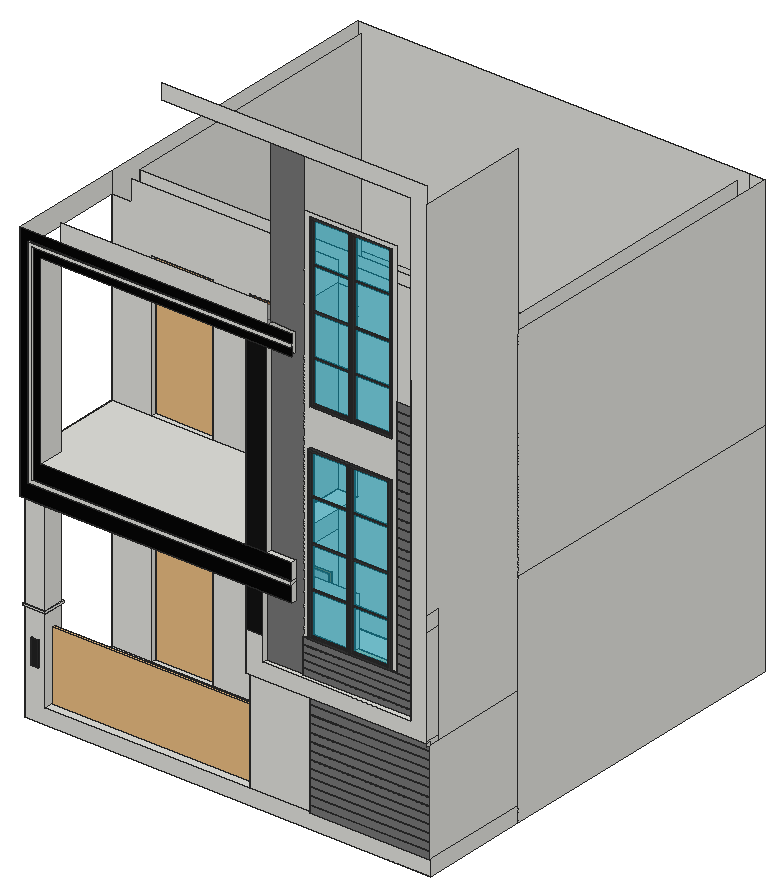
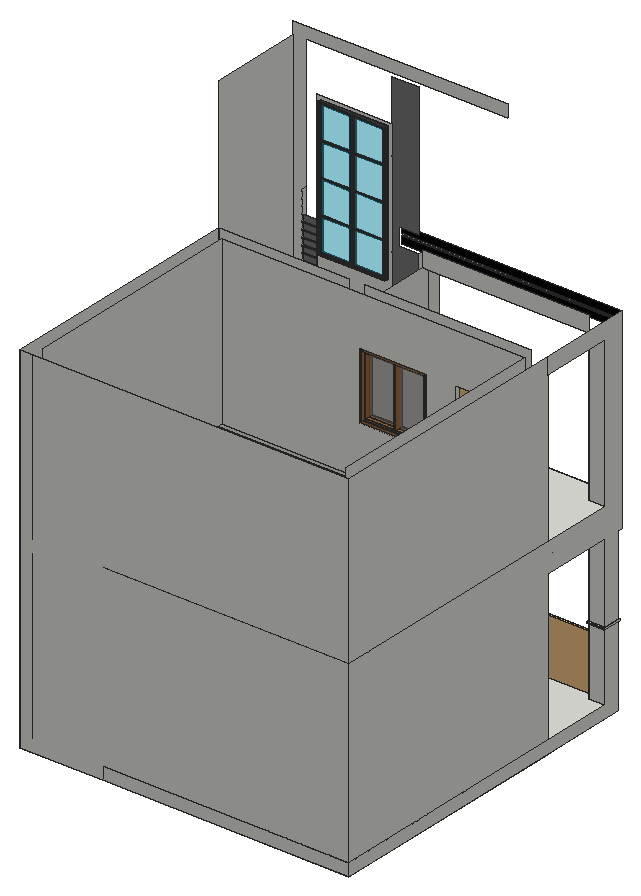
# SketchUp Ruby script. Lengths in inches.
U = 1.inch
M = Sketchup.active_model
def pt(a) = Geom::Point3d.new(a.map { |v| v * U })
def face(e, loops, mat)
  f = e.add_face(loops[0].map { |a| pt(a) })
  loops[1..].each { |l| e.add_face(l.map { |a| pt(a) }).erase! }
  f.material = f.back_material = mat if mat
  f
end
# faces: each face lists its corners as indices into pts; further lists are holes
def faces(e, pts, list, mat = nil) = list.each { |f| face(e, (f[0].is_a?(Array) ? f : [f]).map { |l| l.map { |i| pts[i] } }, mat) }
# xy, xz, yz: faces in a plane at the given z, y or x. An outline is a flat list of corners, or four numbers for a rectangle; further outlines are holes
def ring(l) = l.size == 4 ? [[l[0], l[1]], [l[2], l[1]], [l[2], l[3]], [l[0], l[3]]] : l.each_slice(2).to_a
def flat(e, list, mat, &to3) = list.each { |f| face(e, (f[0].is_a?(Array) ? f : [f]).map { |l| ring(l).map { |u, v| to3.(u, v) } }, mat) }
def xy(e, z, list, mat = nil) = flat(e, list, mat) { |x, y| [x, y, z] }
def xz(e, y, list, mat = nil) = flat(e, list, mat) { |x, z| [x, y, z] }
def yz(e, x, list, mat = nil) = flat(e, list, mat) { |y, z| [x, y, z] }
def lines(e, pts, list) = list.each { |a, b| e.add_line(pt(pts[a]), pt(pts[b])) }
# prism: a flat outline (further loops are holes) pulled along v
def prism(e, loops, v, mat = nil)
  f = face(e, loops, mat); d = Geom::Vector3d.new(v.map { |x| x * U })
  f.pushpull(f.normal.samedirection?(d) ? d.length : -d.length)
end
def box(e, o, s, mat = nil) = prism(e, [[o, [o[0] + s[0], o[1], o[2]], [o[0] + s[0], o[1] + s[1], o[2]], [o[0], o[1] + s[1], o[2]]]], [0, 0, s[2]], mat)
def at(x, y, z, deg = 0) = Geom::Transformation.translation(pt([x, y, z])) * Geom::Transformation.rotation(ORIGIN, Z_AXIS, deg.degrees)
def axes(o, x, y, z) = Geom::Transformation.new([*x, 0, *y, 0, *z, 0, *pt(o).to_a, 1])
def part(name) = M.definitions.add(name)
# library, detail: a bought-in or finely detailed component or shape, given as its bounding box
def library(name, o, s) = part(name).tap { |d| box(d.entities, o, s) }
def detail(e, o, s) = box(e.add_group.entities, o, s)
def put(e, d, t, mat = nil) = e.add_instance(d, t).tap { |i| i.material = mat if mat }
def group(e, t, mat = nil) = e.add_group.tap { |g| g.transformation = t; g.material = mat if mat }.entities
root = M.entities
M.materials.add("[0047_Khaki]").color = [211, 207, 171]
M.materials.add("[0135_DarkGray]1").color = [119, 119, 119]
M.materials.add("[0136_Charcoal]").color = [7, 7, 7]
M.materials.add("[0136_Charcoal]1").color = [20, 20, 20]
M.materials.add("[0136_Charcoal]2").color = [35, 35, 35]
M.materials.add("[Color M07]").color = [58, 58, 58]
M.materials.add("[Translucent Glass Gray]").color = [128, 128, 128]
M.materials["[Translucent Glass Gray]"].alpha = 0.5
M.materials.add("[Translucent Glass Tinted]1").color = [7, 201, 240]
M.materials["[Translucent Glass Tinted]1"].alpha = 0.48
M.materials.add("[Wood Floor]").color = [155, 105, 61]
c1 = library("Louvered terrace screen",[0,0,0],[122,4.25,84])
c2 = library("porta 4",[0.2,-5.42,1.33],[46.55,4.72,83.21])
c3 = part("window full")
xy(c3.entities,0,[[0,0,14.17,66.54]])
xy(c3.entities,2.26,[[12.2,2.26,14.17,64.28]],"[Wood Floor]")
xy(c3.entities,2.36,[[0,2.36,1.97,64.17]],"[Wood Floor]")
xy(c3.entities,3.74,[[11.42,3.74,12.2,32.875],[11.42,33.66,12.2,62.79]],"[Wood Floor]")
xy(c3.entities,3.9375,[[1.97,3.9375,2.76,32.77],[1.97,33.76,2.76,62.6]],"[Wood Floor]")
xy(c3.entities,4.18,[[2.76,4.18,7.09,32.09],[7.09,4.18,11.42,32.09],[2.76,34.45,7.09,62.35],[7.09,34.45,11.42,62.35]],"[Wood Floor]")
xy(c3.entities,69.83,[[2.76,4.18,7.09,32.09],[7.09,32.09,11.42,34.45],[2.76,34.45,7.09,62.35]])
xy(c3.entities,69.83,[[7.09,4.18,11.42,32.09],[7.09,34.45,11.42,62.35]],"[Wood Floor]")
xy(c3.entities,70.08,[[1.97,3.9375,2.76,32.77],[1.97,33.76,2.76,62.6]])
xy(c3.entities,70.27,[[11.42,32.875,12.2,33.66]])
xy(c3.entities,70.27,[[11.42,3.74,12.2,32.875],[11.42,33.66,12.2,62.79]],"[Wood Floor]")
xy(c3.entities,71.65,[[0,2.36,1.97,64.17]])
xy(c3.entities,71.76,[[12.2,2.26,14.17,64.28]],"[Wood Floor]")
xy(c3.entities,74.02,[[0,0,14.17,66.54]],"[Wood Floor]")
xz(c3.entities,0,[[0,0,14.17,74.02]],"[Wood Floor]")
xz(c3.entities,2.26,[[12.2,2.26,14.17,71.76]],"[Wood Floor]")
xz(c3.entities,2.36,[[0,2.36,1.97,71.65]],"[Wood Floor]")
xz(c3.entities,3.74,[[11.42,3.74,12.2,70.27]],"[Wood Floor]")
xz(c3.entities,3.9375,[[1.97,3.9375,2.76,70.08]],"[Wood Floor]")
xz(c3.entities,4.18,[[2.76,4.18,7.09,69.83],[7.09,4.18,11.42,69.83]],"[Wood Floor]")
xz(c3.entities,32.09,[[2.76,4.18,11.42,69.83]],"[Wood Floor]")
xz(c3.entities,32.77,[[1.97,3.9375,2.76,70.08]],"[Wood Floor]")
xz(c3.entities,32.875,[[11.42,3.74,12.2,70.27]],"[Wood Floor]")
xz(c3.entities,33.66,[[11.42,3.74,12.2,47.88],[11.42,47.88,12.2,70.27]],"[Wood Floor]")
xz(c3.entities,33.76,[[1.97,3.9375,2.76,70.08]],"[Wood Floor]")
xz(c3.entities,34.45,[[2.76,4.18,11.42,69.83]],"[Wood Floor]")
xz(c3.entities,62.35,[[2.76,4.18,7.09,69.83],[7.09,4.18,11.42,69.83]],"[Wood Floor]")
xz(c3.entities,62.6,[[1.97,3.9375,2.76,70.08]],"[Wood Floor]")
xz(c3.entities,62.79,[[11.42,3.74,12.2,70.27]],"[Wood Floor]")
xz(c3.entities,64.17,[[0,2.36,1.97,71.65]],"[Wood Floor]")
xz(c3.entities,64.28,[[12.2,2.26,14.17,71.76]],"[Wood Floor]")
xz(c3.entities,66.54,[[0,0,14.17,74.02]],"[Wood Floor]")
yz(c3.entities,0,[[[0,0,66.54,74.02],[2.36,2.36,64.17,71.65]]],"[Wood Floor]")
yz(c3.entities,1.97,[[[2.36,2.36,64.17,71.65],[33.76,3.9375,62.6,70.08],[3.9375,3.9375,32.77,70.08]]],"[Wood Floor]")
yz(c3.entities,2.76,[[32.77,3.9375,33.76,4.18],[32.77,4.18,33.76,69.83],[32.77,69.83,33.76,70.08]])
yz(c3.entities,2.76,[[[3.9375,3.9375,32.77,70.08],[4.18,4.18,32.09,69.83]],[[33.76,3.9375,62.6,70.08],[34.45,4.18,62.35,69.83]]],"[Wood Floor]")
yz(c3.entities,7.09,[[4.18,4.18,62.35,69.83]],"[Translucent Glass Gray]")
yz(c3.entities,11.42,[[32.875,69.83,33.66,70.27]])
yz(c3.entities,11.42,[[[3.74,3.74,32.875,70.27],[4.18,4.18,32.09,69.83]],[[33.66,3.74,62.79,70.27],[34.45,4.18,62.35,69.83]]],"[Wood Floor]")
yz(c3.entities,12.2,[[[2.26,2.26,64.28,71.76],[3.74,3.74,32.875,70.27],[33.66,3.74,62.79,70.27]]],"[Wood Floor]")
yz(c3.entities,14.17,[[[0,0,66.54,74.02],[2.26,2.26,64.28,71.76]]],"[Wood Floor]")
p = [[11.42,32.875,70.27],[11.42,32.875,70.28]]
lines(c3.entities,p,[[0,1]])
c4 = part("Group\#2")
yz(c4.entities,0,[[0,0,20.47,25.2]],"[Translucent Glass Tinted]1")
c5 = part("Untitled")
g1 = group(c5.entities,at(0,0,0))
put(g1,c4,at(1.57,1.57,27.56))
put(g1,c4,at(1.57,1.57,1.57))
put(g1,c4,at(1.57,1.57,53.54))
put(g1,c4,at(1.57,1.57,79.53))
g2 = group(g1,at(0,0,0))
xy(g2,0,[[0,0,2.76,23.62]],"[Color M07]")
xy(g2,1.18,[[0,1.18,1.18,22.44],[1.97,1.18,2.76,22.44]],"[Color M07]")
xy(g2,1.57,[[1.18,1.57,1.97,22.05]],"[Color M07]")
xy(g2,26.77,[[1.18,1.57,1.97,22.05]],"[Color M07]")
xy(g2,27.56,[[1.18,1.57,1.97,22.05]],"[Color M07]")
xy(g2,52.76,[[1.18,1.57,1.97,22.05]],"[Color M07]")
xy(g2,53.54,[[1.18,1.57,1.97,22.05]],"[Color M07]")
xy(g2,78.74,[[1.18,1.57,1.97,22.05]],"[Color M07]")
xy(g2,79.53,[[1.18,1.57,1.97,22.05]],"[Color M07]")
xy(g2,104.72,[[1.18,1.57,1.97,22.05]],"[Color M07]")
xy(g2,105.12,[[0,1.18,1.18,22.44],[1.97,1.18,2.76,22.44]],"[Color M07]")
xy(g2,106.3,[[0,0,2.76,23.62]],"[Color M07]")
xz(g2,0,[[0,0,2.76,106.3]],"[Color M07]")
xz(g2,1.18,[[0,1.18,1.18,105.12],[1.97,1.18,2.76,105.12]],"[Color M07]")
xz(g2,1.57,[[1.18,1.57,1.97,26.77],[1.18,27.56,1.97,52.76],[1.18,53.54,1.97,78.74],[1.18,79.53,1.97,104.72]],"[Color M07]")
xz(g2,22.05,[[1.18,1.57,1.97,26.77],[1.18,27.56,1.97,52.76],[1.18,53.54,1.97,78.74],[1.18,79.53,1.97,104.72]],"[Color M07]")
xz(g2,22.44,[[0,1.18,1.18,105.12],[1.97,1.18,2.76,105.12]],"[Color M07]")
xz(g2,23.62,[[0,0,2.76,106.3]],"[Color M07]")
yz(g2,0,[[[0,0,23.62,106.3],[1.18,1.18,22.44,105.12]]],"[Color M07]")
yz(g2,1.18,[[[1.18,1.18,22.44,105.12],[1.57,79.53,22.05,104.72],[1.57,53.54,22.05,78.74],[1.57,1.57,22.05,26.77],[1.57,27.56,22.05,52.76]]],"[Color M07]")
yz(g2,1.97,[[[1.18,1.18,22.44,105.12],[1.57,79.53,22.05,104.72],[1.57,1.57,22.05,26.77],[1.57,53.54,22.05,78.74],[1.57,27.56,22.05,52.76]]],"[Color M07]")
yz(g2,2.76,[[[0,0,23.62,106.3],[1.18,1.18,22.44,105.12]]],"[Color M07]")
xy(root,-9,[[1,4.125,178.75,64.125],[178.75,4.125,238.75,64.125],[1,64.125,178.75,68.1875],[178.75,64.125,238.75,68.1875],[1,68.1875,178.75,248.1875],
  [178.75,68.1875,238.75,248.1875]])
xy(root,0,[[169.04,3.125,238.75,4.125],[13,4.125,133.04,4.125,133.04,68.1875,1,68.1875,1,16.125,13,16.125],[1,68.1875,1,248.1875,178.75,248.1875,178.75,239.1875,10,239.1875,10,77.1875,24.22,77.1875,24.22,68.1875],[24.22,68.1875,60.22,77.1875],[60.22,68.1875,178.75,77.1875],
  [178.75,68.1875,229.75,77.1875],[10,77.1875,229.75,239.1875],[178.75,239.1875,229.75,248.1875]])
xy(root,4.1875,[[169.04,3.125,238.75,4.125]])
xy(root,4.6875,[[169.04,3.125,238.75,4.125]])
xy(root,9.03,[[169.04,3.125,238.75,4.125]])
xy(root,9.53,[[169.04,3.125,238.75,4.125]])
xy(root,13.72,[[169.04,3.125,238.75,4.125]])
xy(root,14.22,[[169.04,3.125,238.75,4.125]])
xy(root,18.5625,[[169.04,3.125,238.75,4.125]])
xy(root,19.0625,[[169.04,3.125,238.75,4.125]])
xy(root,19.86,[[5.36,3.625,9.3,4.125]],"[0136_Charcoal]2")
xy(root,23.25,[[169.04,3.125,238.75,4.125]])
xy(root,23.75,[[169.04,3.125,238.75,4.125]])
xy(root,28.09,[[169.04,3.125,238.75,4.125]])
xy(root,28.59,[[169.04,3.125,238.75,4.125]])
xy(root,32.78,[[169.04,3.125,238.75,4.125]])
xy(root,33.28,[[169.04,3.125,238.75,4.125]])
xy(root,34.43,[[5.36,3.625,9.3,4.125]],"[0136_Charcoal]2")
xy(root,36,[[81.85,68.1875,129.85,77.1875]])
xy(root,37.625,[[169.04,3.125,238.75,4.125]])
xy(root,38.125,[[169.04,3.125,238.75,4.125]])
xy(root,42.3125,[[169.04,3.125,238.75,4.125]])
xy(root,42.8125,[[169.04,3.125,238.75,4.125]])
xy(root,47.16,[[169.04,3.125,238.75,4.125]])
xy(root,47.66,[[169.04,3.125,238.75,4.125]])
xy(root,49.625,[[0.5,3.6875,13.5,4.125],[0.5,4.125,1,17.4375],[13,4.125,13.5,17.4375],[1,16.125,13,17.4375]])
xy(root,50.625,[[0.5,3.6875,13.5,4.125],[0.5,4.125,1,17.4375],[1,4.125,13,16.125],[13,4.125,13.5,17.4375],[1,16.125,13,17.4375]])
xy(root,51.84,[[169.04,3.125,238.75,4.125]])
xy(root,52.34,[[169.04,3.125,238.75,4.125]])
xy(root,56.6875,[[169.04,3.125,238.75,4.125]])
xy(root,57.1875,[[169.04,3.125,238.75,4.125]])
xy(root,60,[[133.04,10.125,238.75,68.1875]])
xy(root,61.875,[[133.04,1.125,133.04,4.125,169.04,4.125,169.04,3.125,238.75,3.125,238.75,1.125]])
xy(root,70.875,[[143.04,1.125,229.75,1.125,229.75,3.625,164.62,3.625,164.62,4.125,143.04,4.125]])
xy(root,74.45,[[164.62,3.625,229.75,4.125]])
xy(root,74.95,[[164.62,3.625,229.75,4.125]])
xy(root,78.52,[[164.62,3.625,229.75,4.125]])
xy(root,79.02,[[164.62,3.625,229.75,4.125]])
xy(root,82.6,[[164.62,3.625,229.75,4.125]])
xy(root,83.1,[[164.62,3.625,229.75,4.125]])
xy(root,84,[[24.22,68.1875,60.22,77.1875],[81.85,68.1875,129.85,77.1875]])
xy(root,86.67,[[164.62,3.625,229.75,4.125]])
xy(root,90.75,[[164.62,3.625,219.1875,4.125],[219.1875,3.625,229.75,4.125]])
xy(root,91.25,[[219.1875,3.625,229.75,4.125]])
xy(root,91.26,[[191.9,4.125,216.85,10.125]],"[0047_Khaki]")
xy(root,95.82,[[219.1875,3.625,229.75,4.125]])
xy(root,96.32,[[219.1875,3.625,229.75,4.125]])
xy(root,100.9,[[219.1875,3.625,229.75,4.125]])
xy(root,101.4,[[219.1875,3.625,229.75,4.125]])
xy(root,105.97,[[219.1875,3.625,229.75,4.125]])
xy(root,106.47,[[219.1875,3.625,229.75,4.125]])
xy(root,108,[[1,1.125,13,4.125],[13,1.125,133.04,16.125],[143.04,1.125,160.04,4.125]])
xy(root,108.0625,[[1,16.125,12.875,68.1875]])
xy(root,111.05,[[219.1875,3.625,229.75,4.125]])
xy(root,111.55,[[219.1875,3.625,229.75,4.125]])
xy(root,116.125,[[219.1875,3.625,229.75,4.125]])
xy(root,116.625,[[219.1875,3.625,229.75,4.125]])
xy(root,117.5,[[6.5,0.125,160.04,1.125]])
xy(root,119.5,[[8.5,0.125,160.04,1.125]])
xy(root,120,[[12.875,16.125,133.04,64.125],[12.875,64.125,133.04,68.1875],[10,77.1875,178.75,239.1875]])
xy(root,121.2,[[219.1875,3.625,229.75,4.125]])
xy(root,121.7,[[219.1875,3.625,229.75,4.125]])
xy(root,126.27,[[219.1875,3.625,229.75,4.125]])
xy(root,126.77,[[219.1875,3.625,229.75,4.125]])
xy(root,129,[[13,1.125,133.04,1.125,133.04,68.1875,1,68.1875,1,16.125,13,16.125],[145.04,1.125,160.04,4.125],[133.04,10.125,145.04,68.1875],[24.22,68.1875,60.22,77.1875]])
xy(root,131.35,[[219.1875,3.625,229.75,4.125]])
xy(root,131.85,[[219.1875,3.625,229.75,4.125]])
xy(root,136.42,[[219.1875,3.625,229.75,4.125]])
xy(root,136.92,[[219.1875,3.625,229.75,4.125]])
xy(root,141.5,[[219.1875,3.625,229.75,4.125]])
xy(root,142,[[219.1875,3.625,229.75,4.125]])
xy(root,146.57,[[219.1875,3.625,229.75,4.125]])
xy(root,147.07,[[219.1875,3.625,229.75,4.125]])
xy(root,151.65,[[219.1875,3.625,229.75,4.125]])
xy(root,152.15,[[219.1875,3.625,229.75,4.125]])
xy(root,156.73,[[219.1875,3.625,229.75,4.125]])
xy(root,157.23,[[219.1875,3.625,229.75,4.125]])
xy(root,161.8,[[219.1875,3.625,229.75,4.125]])
xy(root,162.3,[[219.1875,3.625,229.75,4.125]])
xy(root,165,[[81.85,68.1875,129.85,77.1875]])
xy(root,166.875,[[219.1875,3.625,229.75,4.125]])
xy(root,167.375,[[219.1875,3.625,229.75,4.125]])
xy(root,171.95,[[219.1875,3.625,229.75,4.125]])
xy(root,172.45,[[219.1875,3.625,229.75,4.125]])
xy(root,177.03,[[219.1875,3.625,229.75,4.125]])
xy(root,177.53,[[219.1875,3.625,229.75,4.125]])
xy(root,182.1,[[219.1875,3.625,229.75,4.125]])
xy(root,182.6,[[219.1875,3.625,229.75,4.125]])
xy(root,187.18,[[219.1875,3.625,229.75,4.125]])
xy(root,187.68,[[219.1875,3.625,229.75,4.125]])
xy(root,192.25,[[219.1875,3.625,229.75,4.125]])
xy(root,192.75,[[219.1875,3.625,229.75,4.125]])
xy(root,197.33,[[219.1875,3.625,229.75,4.125]])
xy(root,197.83,[[219.1875,3.625,229.75,4.125]])
xy(root,202.4,[[219.1875,3.625,229.75,4.125]])
xy(root,202.9,[[219.1875,3.625,229.75,4.125]])
xy(root,207.48,[[219.1875,3.625,229.75,4.125]])
xy(root,207.98,[[219.1875,3.625,229.75,4.125]])
xy(root,212.55,[[219.1875,3.625,229.75,4.125]])
xy(root,213,[[24.22,68.1875,60.22,77.1875],[81.85,68.1875,129.85,77.1875]])
xy(root,213.05,[[219.1875,3.625,229.75,4.125]])
xy(root,217.625,[[219.1875,3.625,229.75,4.125]])
xy(root,218.125,[[219.1875,3.625,229.75,4.125]])
xy(root,222.7,[[219.1875,3.625,229.75,4.125]])
xy(root,223.2,[[219.1875,3.625,229.75,4.125]])
xy(root,227.78,[[219.1875,3.625,229.75,4.125]])
xy(root,228.28,[[219.1875,3.625,229.75,4.125]])
xz(root,0.125,[[6.5,117.5,160.04,117.5,160.04,119.5,8.5,119.5,8.5,242,160.04,242,160.04,244,6.5,244]])
xz(root,1.125,[[133.04,61.875,238.75,61.875,238.75,354,83.7,354,83.7,345,229.75,345,229.75,70.875,143.04,70.875,143.04,84.9375,133.04,84.9375]])
xz(root,1.125,[[1,108,160.04,108,160.04,117.5,6.5,117.5,6.5,244,160.04,244,160.04,249,1,249],[8.5,119.5,160.04,119.5,160.04,129,13,129,13,237,160.04,237,160.04,242,8.5,242]],"[0136_Charcoal]")
xz(root,1.125,[[133.04,84.9375,143.04,108],[133.04,129,145.04,237]],"[0136_Charcoal]1")
xz(root,3.125,[[169.04,0,238.75,4.1875],[169.04,4.6875,238.75,9.03],[169.04,9.53,238.75,13.72],[169.04,14.22,238.75,18.5625],[169.04,19.0625,238.75,23.25],
  [169.04,23.75,238.75,28.09],[169.04,28.59,238.75,32.78],[169.04,33.28,238.75,37.625],[169.04,38.125,238.75,42.3125],[169.04,42.8125,238.75,47.16],
  [169.04,47.66,238.75,51.84],[169.04,52.34,238.75,56.6875],[169.04,57.1875,238.75,61.875]],"[0135_DarkGray]1")
xz(root,3.625,[[164.62,70.875,229.75,74.45],[164.62,74.95,229.75,78.52],[164.62,79.02,229.75,82.6],[164.62,83.1,229.75,86.67],[164.62,87.18,229.75,90.75],
  [219.1875,91.25,229.75,95.82],[219.1875,96.32,229.75,100.9],[219.1875,101.4,229.75,105.97],[219.1875,106.47,229.75,111.05],[219.1875,111.55,229.75,116.125],
  [219.1875,116.625,229.75,121.2],[219.1875,121.7,229.75,126.27],[219.1875,126.77,229.75,131.35],[219.1875,131.85,229.75,136.42],[219.1875,136.92,229.75,141.5],
  [219.1875,142,229.75,146.57],[219.1875,147.07,229.75,151.65],[219.1875,152.15,229.75,156.73],[219.1875,157.23,229.75,161.8],[219.1875,162.3,229.75,166.875],
  [219.1875,167.375,229.75,171.95],[219.1875,172.45,229.75,177.03],[219.1875,177.53,229.75,182.1],[219.1875,182.6,229.75,187.18],[219.1875,187.68,229.75,192.25],
  [219.1875,192.75,229.75,197.33],[219.1875,197.83,229.75,202.4],[219.1875,202.9,229.75,207.48],[219.1875,207.98,229.75,212.55],[219.1875,213.05,229.75,217.625],
  [219.1875,218.125,229.75,222.7],[219.1875,223.2,229.75,227.78],[219.1875,228.28,229.75,232.85]],"[0135_DarkGray]1")
xz(root,3.625,[[5.36,19.86,9.3,34.43]],"[0136_Charcoal]2")
xz(root,3.6875,[[0.5,49.625,13.5,50.625]])
xz(root,4.125,[[[1,-9,238.75,-9,238.75,0,13,0,13,49.625,1,49.625],[5.36,19.86,9.3,34.43]],[133.04,0,169.04,61.875],[169.04,4.1875,238.75,4.6875],[169.04,9.03,238.75,9.53],[169.04,13.72,238.75,14.22],
  [169.04,18.5625,238.75,19.0625],[169.04,23.25,238.75,23.75],[169.04,28.09,238.75,28.59],[169.04,32.78,238.75,33.28],[169.04,37.625,238.75,38.125],
  [169.04,42.3125,238.75,42.8125],[169.04,47.16,238.75,47.66],[1,50.625,13,108],[169.04,51.84,238.75,52.34],[169.04,56.6875,238.75,57.1875],
  [164.62,74.45,229.75,74.95],[164.62,78.52,229.75,79.02],[164.62,82.6,229.75,83.1],[164.62,86.67,229.75,87.17],[164.62,90.75,229.75,91.25],
  [[164.62,91.25,191.9,91.25,191.9,91.26,167.92,91.26,167.92,191.2,216.85,191.2,216.85,91.26,191.9,91.26,191.9,91.25,219.1875,91.25,219.1875,314.55,164.62,314.55],[167.92,212.2,216.85,312.13]],[219.1875,95.82,229.75,96.32],[219.1875,100.9,229.75,101.4],[219.1875,105.97,229.75,106.47],[219.1875,111.05,229.75,111.55],
  [219.1875,116.125,229.75,116.625],[219.1875,121.2,229.75,121.7],[219.1875,126.27,229.75,126.77],[219.1875,131.35,229.75,131.85],[219.1875,136.42,229.75,136.92],
  [219.1875,141.5,229.75,142],[219.1875,146.57,229.75,147.07],[219.1875,151.65,229.75,152.15],[219.1875,156.73,229.75,157.23],[219.1875,161.8,229.75,162.3],
  [219.1875,166.875,229.75,167.375],[219.1875,171.95,229.75,172.45],[219.1875,177.03,229.75,177.53],[219.1875,182.1,229.75,182.6],[219.1875,187.18,229.75,187.68],
  [219.1875,192.25,229.75,192.75],[219.1875,197.33,229.75,197.83],[219.1875,202.4,229.75,202.9],[219.1875,207.48,229.75,207.98],[219.1875,212.55,229.75,213.05],
  [219.1875,217.625,229.75,218.125],[219.1875,222.7,229.75,223.2],[219.1875,227.78,229.75,228.28]])
xz(root,4.125,[[143.04,70.875,164.62,70.875,164.62,345,145.04,345,145.04,249,160.04,249,160.04,237,145.04,237,145.04,129,160.04,129,160.04,108,143.04,108]],"[0135_DarkGray]1")
xz(root,10.125,[[133.04,60,238.75,62.69],[133.04,62.69,133.04,120,191.9,120,191.9,91.26,216.85,91.26,216.85,120,238.75,120,238.75,62.69]])
xz(root,16.125,[[1,0,13,49.625],[1,50.625,1,108.0625,12.875,108.0625,12.875,120,133.04,120,133.04,108,13,108,13,50.625],[1,129,1,237.0625,12.875,237.0625,12.875,249,133.04,249,133.04,237,13,237,13,129]])
xz(root,17.4375,[[0.5,49.625,13.5,50.625]])
xz(root,68.1875,[[[1,0,24.22,0,24.22,84,60.22,84,60.22,0,133.04,0,133.04,120,12.875,120,12.875,108.0625,1,108.0625],[81.85,36,129.85,84]],[133.04,0,238.75,60],[133.04,60,238.75,120],[133.04,120,238.75,120,238.75,249,145.04,249,145.04,129,133.04,129],[[1,129,24.22,129,24.22,213,60.22,213,60.22,129,133.04,129,133.04,249,12.875,249,12.875,237.0625,1,237.0625],[81.85,165,129.85,213]],
  [133.04,129,145.04,237]])
xz(root,77.1875,[[[10,0,10,120,229.75,120,229.75,0,60.22,0,60.22,84,24.22,84,24.22,0],[81.85,36,129.85,84]],[[10,129,10,249,229.75,249,229.75,129,60.22,129,60.22,213,24.22,213,24.22,129],[81.85,165,129.85,213]]])
xz(root,248.1875,[[1,-9,178.75,0],[178.75,-9,178.75,0,1,0,1,249,238.75,249,238.75,-9]])
yz(root,0.5,[[3.6875,49.625,17.4375,50.625]])
yz(root,1,[[4.125,-9,4.125,49.625,16.125,49.625,16.125,0,248.1875,0,248.1875,-9],[68.1875,0,68.1875,108.0625,16.125,108.0625,16.125,50.625,4.125,50.625,4.125,108,1.125,108,1.125,249,68.1875,249,68.1875,237.0625,16.125,237.0625,16.125,129,248.1875,129,248.1875,0],[68.1875,129,248.1875,249]])
yz(root,5.36,[[3.625,19.86,4.125,34.43]],"[0136_Charcoal]2")
yz(root,6.5,[[0.125,117.5,1.125,244]])
yz(root,8.5,[[0.125,119.5,1.125,242]])
yz(root,9.3,[[3.625,19.86,4.125,34.43]],"[0136_Charcoal]2")
yz(root,10,[[77.1875,0,239.1875,120],[77.1875,129,239.1875,249]])
yz(root,12.875,[[16.125,108.0625,68.1875,120]])
yz(root,13,[[4.125,0,16.125,49.625],[4.125,50.625,16.125,108],[1.125,129,16.125,237]])
yz(root,13.5,[[3.6875,49.625,17.4375,50.625]])
yz(root,24.22,[[68.1875,0,77.1875,84],[68.1875,129,77.1875,213]])
yz(root,60.22,[[68.1875,0,77.1875,84],[68.1875,129,77.1875,213]])
yz(root,81.85,[[68.1875,36,77.1875,84],[68.1875,165,77.1875,213]])
yz(root,129.85,[[68.1875,36,77.1875,84],[68.1875,165,77.1875,213]])
yz(root,133.04,[[4.125,0,4.125,61.875,1.125,61.875,1.125,108,10.125,108,10.125,60,68.1875,60,68.1875,0],[10.125,108,16.125,108,16.125,120,68.1875,120,68.1875,129,10.125,129],[16.125,108,68.1875,120],[1.125,129,10.125,237],[10.125,129,68.1875,237]])
yz(root,143.04,[[1.125,70.875,4.125,108]])
yz(root,145.04,[[1.125,129,4.125,237]])
yz(root,160.04,[[1.125,108,4.125,117.5],[0.125,117.5,4.125,119.5],[1.125,119.5,4.125,129]])
yz(root,164.62,[[3.625,70.875,4.125,74.45],[3.625,74.95,4.125,78.52],[3.625,79.02,4.125,82.6],[3.625,83.1,4.125,86.67],[4.125,87.17,3.625,87.18,3.625,90.75,4.125,90.75]])
yz(root,169.04,[[3.125,0,4.125,4.1875],[3.125,4.6875,4.125,9.03],[3.125,9.53,4.125,13.72],[3.125,14.22,4.125,18.5625],[3.125,19.0625,4.125,23.25],
  [3.125,23.75,4.125,28.09],[3.125,28.59,4.125,32.78],[3.125,33.28,4.125,37.625],[3.125,38.125,4.125,42.3125],[3.125,42.8125,4.125,47.16],
  [3.125,47.66,4.125,51.84],[3.125,52.34,4.125,56.6875],[3.125,57.1875,4.125,61.875]])
yz(root,219.1875,[[3.625,91.25,4.125,95.82],[3.625,96.32,4.125,100.9],[3.625,101.4,4.125,105.97],[3.625,106.47,4.125,111.05],[3.625,111.55,4.125,116.125],
  [3.625,116.625,4.125,121.2],[3.625,121.7,4.125,126.27],[3.625,126.77,4.125,131.35],[3.625,131.85,4.125,136.42],[3.625,136.92,4.125,141.5],
  [3.625,142,4.125,146.57],[3.625,147.07,4.125,151.65],[3.625,152.15,4.125,156.73],[3.625,157.23,4.125,161.8],[3.625,162.3,4.125,166.875],
  [3.625,167.375,4.125,171.95],[3.625,172.45,4.125,177.03],[3.625,177.53,4.125,182.1],[3.625,182.6,4.125,187.18],[3.625,187.68,4.125,192.25],
  [3.625,192.75,4.125,197.33],[3.625,197.83,4.125,202.4],[3.625,202.9,4.125,207.48],[3.625,207.98,4.125,212.55],[3.625,213.05,4.125,217.625],
  [3.625,218.125,4.125,222.7],[3.625,223.2,4.125,227.78],[3.625,228.28,4.125,232.85]])
yz(root,229.75,[[77.1875,0,239.1875,120],[1.125,70.875,1.125,129,3.625,129,3.625,126.77,4.125,126.77,4.125,126.27,3.625,126.27,3.625,121.7,4.125,121.7,4.125,121.2,3.625,121.2,3.625,116.625,4.125,116.625,4.125,116.125,3.625,116.125,3.625,111.55,4.125,111.55,4.125,111.05,3.625,111.05,3.625,106.47,4.125,106.47,4.125,105.97,3.625,105.97,3.625,101.4,4.125,101.4,4.125,100.9,3.625,100.9,3.625,96.32,4.125,96.32,4.125,95.82,3.625,95.82,3.625,91.25,4.125,91.25,4.125,90.75,3.625,90.75,3.625,87.18,4.125,87.17,4.125,86.67,3.625,86.67,3.625,83.1,4.125,83.1,4.125,82.6,3.625,82.6,3.625,79.02,4.125,79.02,4.125,78.52,3.625,78.52,3.625,74.95,4.125,74.95,4.125,74.45,3.625,74.45,3.625,70.875],[1.125,129,1.125,249,3.625,249,3.625,248.58,4.125,248.58,4.125,248.08,3.625,248.08,3.625,243.5,4.125,243.5,4.125,243,3.625,243,3.625,238.43,4.125,238.43,4.125,237.93,3.625,237.93,3.625,233.35,4.125,233.35,4.125,232.85,3.625,232.85,3.625,228.28,4.125,228.28,4.125,227.78,3.625,227.78,3.625,223.2,4.125,223.2,4.125,222.7,3.625,222.7,3.625,218.125,4.125,218.125,4.125,217.625,3.625,217.625,3.625,213.05,4.125,213.05,4.125,212.55,3.625,212.55,3.625,207.98,4.125,207.98,4.125,207.48,3.625,207.48,3.625,202.9,4.125,202.9,4.125,202.4,3.625,202.4,3.625,197.83,4.125,197.83,4.125,197.33,3.625,197.33,3.625,192.75,4.125,192.75,4.125,192.25,3.625,192.25,3.625,187.68,4.125,187.68,4.125,187.18,3.625,187.18,3.625,182.6,4.125,182.6,4.125,182.1,3.625,182.1,3.625,177.53,4.125,177.53,4.125,177.03,3.625,177.03,3.625,172.45,4.125,172.45,4.125,171.95,3.625,171.95,3.625,167.375,4.125,167.375,4.125,166.875,3.625,166.875,3.625,162.3,4.125,162.3,4.125,161.8,3.625,161.8,3.625,157.23,4.125,157.23,4.125,156.73,3.625,156.73,3.625,152.15,4.125,152.15,4.125,151.65,3.625,151.65,3.625,147.07,4.125,147.07,4.125,146.57,3.625,146.57,3.625,142,4.125,142,4.125,141.5,3.625,141.5,3.625,136.92,4.125,136.92,4.125,136.42,3.625,136.42,3.625,131.85,4.125,131.85,4.125,131.35,3.625,131.35,3.625,129],[77.1875,129,239.1875,249]])
yz(root,238.75,[[4.125,-9,68.1875,0],[68.1875,-9,248.1875,120],[3.125,0,68.1875,0,68.1875,60,3.125,60,3.125,57.1875,4.125,57.1875,4.125,56.6875,3.125,56.6875,3.125,52.34,4.125,52.34,4.125,51.84,3.125,51.84,3.125,47.66,4.125,47.66,4.125,47.16,3.125,47.16,3.125,42.8125,4.125,42.8125,4.125,42.3125,3.125,42.3125,3.125,38.125,4.125,38.125,4.125,37.625,3.125,37.625,3.125,33.28,4.125,33.28,4.125,32.78,3.125,32.78,3.125,28.59,4.125,28.59,4.125,28.09,3.125,28.09,3.125,23.75,4.125,23.75,4.125,23.25,3.125,23.25,3.125,19.0625,4.125,19.0625,4.125,18.5625,3.125,18.5625,3.125,14.22,4.125,14.22,4.125,13.72,3.125,13.72,3.125,9.53,4.125,9.53,4.125,9.03,3.125,9.03,3.125,4.6875,4.125,4.6875,4.125,4.1875,3.125,4.1875],[1.125,60,3.125,61.875],[10.125,60,68.1875,60,68.1875,344.33,1.125,344.33,1.125,129,10.125,129],
  [3.125,60,10.125,60,10.125,62.69,1.125,62.69,1.125,61.875,3.125,61.875],[1.125,62.69,10.125,120],[1.125,120,10.125,129],[68.1875,120,248.1875,249]])
p = [[164.62,4.125,87.17],[229.75,4.125,87.17],[229.75,3.625,87.18],[164.62,3.625,87.18],[229.75,248.1875,0],[229.75,248.1875,120],
  [229.75,248.1875,129],[229.75,248.1875,249],[229.75,4.125,129],[229.75,10.125,129],[178.75,248.1875,129],[1,248.1875,129],
  [178.75,239.1875,129],[10,239.1875,129],[145.04,4.125,129],[145.04,10.125,129],[1,64.125,120],[12.875,64.125,120],
  [178.75,77.1875,120],[178.75,68.1875,120],[229.75,4.125,79.02],[231,4.125,79.02],[192.39,4.125,212.2],[192.39,4.125,312.13],
  [192.39,4.125,191.2],[191.9,4.125,91.26]]
faces(root,p,[[0,1,2,3]])
lines(root,p,[[4,5],[6,7],[8,9],[10,11],[12,13],[14,15],[16,17],[18,19],[20,21],[22,23],[24,25]])
put(root,c1,axes([12,9.08,0],[0.99211,0,0],[0,0.48,0],[0,0,0.48]))
put(root,c2,axes([24.07,75.1,-1.34],[0.77339,0,0],[0,0.752,0],[0,0,1.00712]))
put(root,c3,axes([81.85,77.08,36],[0,-0.62,0],[0.7192,0,0],[0,0,0.65137]))
put(root,c5,axes([192.0625,2.78,91.26],[0,0.93771,0],[-1.0221,0,0],[0,0,0.93771]))
put(root,c5,axes([216.21,2.78,91.26],[0,0.93771,0],[-1.0221,0,0],[0,0,0.93771]))
put(root,c2,axes([24.07,75.1,127.66],[0.77339,0,0],[0,0.752,0],[0,0,1.00712]))
put(root,c3,axes([81.85,77.08,165],[0,-0.62,0],[0.7192,0,0],[0,0,0.65137]))
put(root,c5,axes([216.21,4.125,212.2],[0,0.93771,0],[-1.0221,0,0],[0,0,0.93771]))
put(root,c5,axes([192.0625,4.125,212.2],[0,0.93771,0],[-1.0221,0,0],[0,0,0.93771]))
